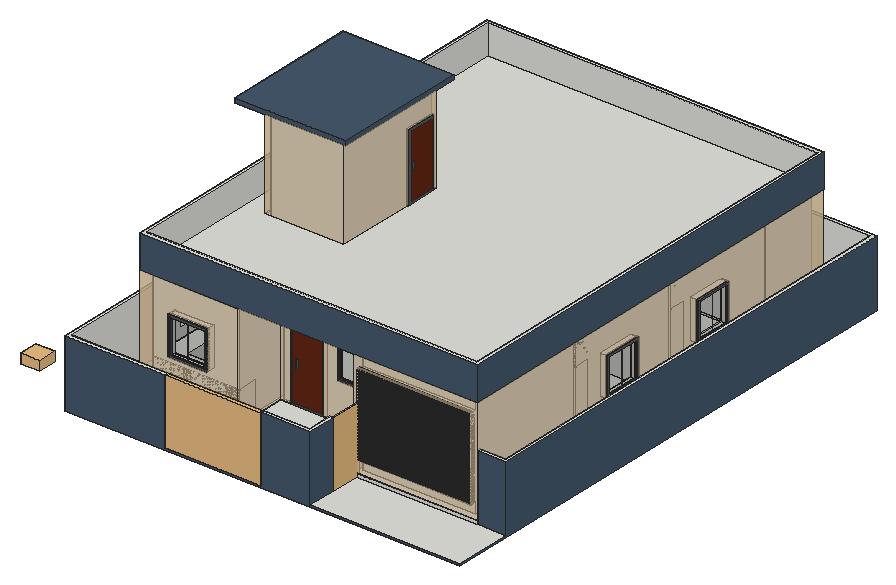
# SketchUp Ruby script. Lengths in inches.
U = 1.inch
M = Sketchup.active_model
def pt(a) = Geom::Point3d.new(a.map { |v| v * U })
def face(e, loops, mat)
  f = e.add_face(loops[0].map { |a| pt(a) })
  loops[1..].each { |l| e.add_face(l.map { |a| pt(a) }).erase! }
  f.material = f.back_material = mat if mat
  f
end
# faces: each face lists its corners as indices into pts; further lists are holes
def faces(e, pts, list, mat = nil) = list.each { |f| face(e, (f[0].is_a?(Array) ? f : [f]).map { |l| l.map { |i| pts[i] } }, mat) }
# xy, xz, yz: faces in a plane at the given z, y or x. An outline is a flat list of corners, or four numbers for a rectangle; further outlines are holes
def ring(l) = l.size == 4 ? [[l[0], l[1]], [l[2], l[1]], [l[2], l[3]], [l[0], l[3]]] : l.each_slice(2).to_a
def flat(e, list, mat, &to3) = list.each { |f| face(e, (f[0].is_a?(Array) ? f : [f]).map { |l| ring(l).map { |u, v| to3.(u, v) } }, mat) }
def xy(e, z, list, mat = nil) = flat(e, list, mat) { |x, y| [x, y, z] }
def xz(e, y, list, mat = nil) = flat(e, list, mat) { |x, z| [x, y, z] }
def yz(e, x, list, mat = nil) = flat(e, list, mat) { |y, z| [x, y, z] }
def lines(e, pts, list) = list.each { |a, b| e.add_line(pt(pts[a]), pt(pts[b])) }
# prism: a flat outline (further loops are holes) pulled along v
def prism(e, loops, v, mat = nil)
  f = face(e, loops, mat); d = Geom::Vector3d.new(v.map { |x| x * U })
  f.pushpull(f.normal.samedirection?(d) ? d.length : -d.length)
end
def box(e, o, s, mat = nil) = prism(e, [[o, [o[0] + s[0], o[1], o[2]], [o[0] + s[0], o[1] + s[1], o[2]], [o[0], o[1] + s[1], o[2]]]], [0, 0, s[2]], mat)
def at(x, y, z, deg = 0) = Geom::Transformation.translation(pt([x, y, z])) * Geom::Transformation.rotation(ORIGIN, Z_AXIS, deg.degrees)
def axes(o, x, y, z) = Geom::Transformation.new([*x, 0, *y, 0, *z, 0, *pt(o).to_a, 1])
def part(name) = M.definitions.add(name)
# library, detail: a bought-in or finely detailed component or shape, given as its bounding box
def library(name, o, s) = part(name).tap { |d| box(d.entities, o, s) }
def detail(e, o, s) = box(e.add_group.entities, o, s)
def put(e, d, t, mat = nil) = e.add_instance(d, t).tap { |i| i.material = mat if mat }
def group(e, t, mat = nil) = e.add_group.tap { |g| g.transformation = t; g.material = mat if mat }.entities
root = M.entities
M.materials.add("Chocolate White 001").color = [230, 202, 161]
M.materials["Chocolate White 001"].alpha = 0.6
M.materials.add("Glass Red 001").color = [0, 0, 0]
M.materials["Glass Red 001"].alpha = 0.1
M.materials.add("Metal Sandblasted Black 200cm").color = [86, 90, 95]
M.materials.add("Wall Paint Simple Reflective").color = [70, 89, 109]
M.materials.add("Wood Dark 02 100cm").color = [99, 39, 19]
M.materials.add("[Metal_Aluminum_Anodized]").color = [232, 200, 107]
c1 = library("gate 189k",[0,0,0],[125.98,4.8,118.11])
c2 = library("gate 130k",[0,-0.99,0],[39.37,1.78,88.58])
c3 = library("Dome Light",[-12,-12,0],[24,24,12])
c4 = part("Group\#3")
box(c4.entities,[-0.31,0,0],[0.31,22,44])
c5 = part("Group\#5")
box(c5.entities,[0,-0.31,0],[22,0.31,44])
c6 = part("Group\#13")
box(c6.entities,[0,0,0],[0.31,16,44])
c7 = part("Group\#15")
box(c7.entities,[0,0,0],[0.31,16.32,44])
c8 = part("Group\#19")
box(c8.entities,[0,0,0],[22,0.31,44])
c9 = part("Group\#7")
box(c9.entities,[0,-0.31,0],[32,0.31,2])
c10 = part("Group\#101")
box(c10.entities,[0,0,0],[0.31,22,44])
c11 = part("Group\#11")
box(c11.entities,[0,0,0],[0.31,32,2])
c12 = part("Group\#46")
box(c12.entities,[0,0,0],[0.71,39.5,117.71])
c13 = part("Group\#49")
box(c13.entities,[0,0,0],[0.71,20.65,34.58])
c14 = part("Group\#51")
g1 = group(c14.entities,at(12,0,0))
xy(g1,0,[[-12,0,0,84]])
xy(g1,1.96,[[-12,2.5,-2,81.5]])
xy(g1,94.04,[[-12,2.5,-2,81.5]])
xy(g1,96,[[-12,0,0,84]])
xz(g1,0,[[-12,0,0,96]])
xz(g1,2.5,[[-12,1.96,-2,94.04]])
xz(g1,81.5,[[-12,1.96,-2,94.04]])
xz(g1,84,[[-12,0,0,96]])
yz(g1,-12,[[[0,0,84,96],[2.5,1.96,81.5,94.04]]])
yz(g1,-2,[[2.5,1.96,81.5,94.04]])
yz(g1,0,[[0,0,84,96]])
put(g1,c12,axes([-12,42,1.96],[1,0,0],[0,1,0],[0,0,0.78232]))
put(g1,c12,axes([-12,2.5,1.96],[1,0,0],[0,1,0],[0,0,0.78232]))
g2 = group(c14.entities,at(0,0,96))
box(g2,[0,0,0],[12,84,36])
g3 = group(g2,at(0,21.05,0.71))
box(g3,[0,0,0],[0.71,20.95,34.58])
put(g2,c13,at(0,62.65,0.71))
put(g2,c13,at(0,42,0.71))
g4 = group(g2,at(0,0.1,0.71))
box(g4,[0,0,0],[0.71,20.95,34.58])
c15 = part("Group\#55")
box(c15.entities,[0,0,0],[12,36,6.5625])
c16 = part("Group\#64")
box(c16.entities,[0,0,0],[12,39.5,6.5625])
c17 = part("Group\#57")
box(c17.entities,[0,0,0],[12,36,6])
prism(root,[[[45,190,0],[69,190,0],[69,105,0],[153,105,0],[153,81,0],[45,81,0]]],[0,0,36])
prism(root,[[[45,454.5,0],[153,454.5,0],[153,430.5,0],[69,430.5,0],[69,370.5,0],[45,370.5,0]]],[0,0,36])
put(root,c1,axes([124.8,0,-4],[0.9476,0,0],[0,0.87,0],[0,0,0.69427]))
put(root,c2,axes([305.43,36,-4],[0,0.97964,0],[-1,0,0],[0,0,0.92569]),"[Metal_Aluminum_Anodized]")
put(root,c3,at(-71.79,47.18,1.82))
g5 = group(root,at(36,72,0))
xy(g5,0,[[[0,0,0,540,420,540,420,0,265.5,0,265.5,67,175.5,67,175.5,71.5,265.5,71.5,265.5,260,270,260,270,164,411,164,411,308,270,308,270,296,265.5,296,265.5,324.5,270,324.5,270,312.5,411,312.5,411,456.5,363,456.5,363,461,411,461,411,531,294,531,294,461,327,461,327,456.5,270,456.5,270,360.5,265.5,360.5,265.5,461,289.5,461,289.5,531,157.5,531,157.5,461,229.5,461,229.5,456.5,157.5,456.5,157.5,447,153,447,153,531,9,531,9,387,153,387,153,399,157.5,399,157.5,294,141,294,141,298.5,153,298.5,153,382.5,9,382.5,9,298.5,105,298.5,105,294,9,294,9,158.5,121.5,158.5,121.5,142,117,142,117,154,9,154,9,9,117,9,117,106,121.5,106,121.5,71.5,133.5,71.5,133.5,67,121.5,67,121.5,0],[270,9,411,159.5]]])
xy(g5,15.1875,[[270,0,411,9]])
xy(g5,36,[[270,99.5,294,99.5,294,135.5,387,135.5,387,99.5,411,99.5,411,159.5,270,159.5]])
xy(g5,48,[[36,0,84,9],[0,51.1875,9,99.1875],[193.375,67,241.375,71.5],[0,158.5,9,195.14],[411,201.4375,420,249.4375],
  [0,258,9,294],[411,342.15,420,390.15],[0,430.8125,9,478.8125],[64.4375,531,112.4375,540]])
xy(g5,72,[[0,324.8125,9,360.8125],[210.8125,531,246.8125,540],[339.375,531,375.375,540]])
xy(g5,96,[[36,0,84,9],[0,51.1875,9,99.1875],[133.5,67,175.5,71.5],[193.375,67,241.375,71.5],[117,106,121.5,142],
  [0,158.5,9,195.14],[411,201.4375,420,249.4375],[0,258,9,294],[265.5,260,270,296],[105,294,141,298.5],
  [265.5,324.5,270,360.5],[0,324.8125,9,360.8125],[411,342.15,420,390.15],[153,399,157.5,447],[0,430.8125,9,478.8125],
  [229.5,456.5,265.5,461],[327,456.5,363,461],[64.4375,531,112.4375,540],[210.8125,531,246.8125,540],[339.375,531,375.375,540]])
xy(g5,116.08,[[270,0,411,9]])
xy(g5,132,[[[0,0,121.5,0,121.5,67,265.5,67,265.5,0,420,0,420,540,0,540],[121.5,71.5,121.5,158.5,9,158.5,9,294,157.5,294,157.5,456.5,265.5,456.5,265.5,71.5],[270,9,411,159.5],[9,387,153,531],[270,164,411,308],[270,312.5,411,456.5],[9,9,117,154],[9,298.5,153,382.5],[157.5,461,289.5,531],[294,461,411,531]]])
xz(g5,0,[[[0,0,121.5,132],[36,48,84,96]],[[265.5,0,420,132],[270,15.1875,411,116.08]]],"Chocolate White 001")
xz(g5,9,[[[9,0,117,132],[36,48,84,96]],[270,0,411,15.1875],[270,116.08,411,132]])
xz(g5,51.1875,[[0,48,9,96]])
xz(g5,67,[[[121.5,0,133.5,0,133.5,96,175.5,96,175.5,0,265.5,0,265.5,132,121.5,132],[193.375,48,241.375,96]]],"Chocolate White 001")
xz(g5,71.5,[[[121.5,0,121.5,132,265.5,132,265.5,0,175.5,0,175.5,96,133.5,96,133.5,0],[193.375,48,241.375,96]]])
xz(g5,99.1875,[[0,48,9,96]])
xz(g5,99.5,[[270,0,294,36],[387,0,411,36]])
xz(g5,106,[[117,0,121.5,96]])
xz(g5,135.5,[[294,0,387,36]])
xz(g5,142,[[117,0,121.5,96]])
xz(g5,154,[[9,0,117,132]])
xz(g5,158.5,[[9,0,9,48,0,48,0,96,9,96,9,132,121.5,132,121.5,0]])
xz(g5,159.5,[[270,0,411,36],[270,36,411,132]])
xz(g5,164,[[270,0,411,132]])
xz(g5,195.14,[[0,48,9,96]])
xz(g5,201.4375,[[411,48,420,96]])
xz(g5,249.4375,[[411,48,420,96]])
xz(g5,258,[[0,48,9,96]])
xz(g5,260,[[265.5,0,270,96]])
xz(g5,294,[[9,0,105,0,105,96,141,96,141,0,157.5,0,157.5,132,9,132,9,96,0,96,0,48,9,48]])
xz(g5,296,[[265.5,0,270,96]])
xz(g5,298.5,[[9,0,9,132,153,132,153,0,141,0,141,96,105,96,105,0]])
xz(g5,308,[[270,0,411,132]])
xz(g5,312.5,[[270,0,411,132]])
xz(g5,324.5,[[265.5,0,270,96]])
xz(g5,324.8125,[[0,72,9,96]])
xz(g5,342.15,[[411,48,420,96]])
xz(g5,360.5,[[265.5,0,270,96]])
xz(g5,360.8125,[[0,72,9,96]])
xz(g5,382.5,[[9,0,153,132]])
xz(g5,387,[[9,0,153,132]])
xz(g5,390.15,[[411,48,420,96]])
xz(g5,399,[[153,0,157.5,96]])
xz(g5,430.8125,[[0,48,9,96]])
xz(g5,447,[[153,0,157.5,96]])
xz(g5,456.5,[[157.5,0,229.5,0,229.5,96,265.5,96,265.5,132,157.5,132],[270,0,327,0,327,96,363,96,363,0,411,0,411,132,270,132]])
xz(g5,461,[[157.5,0,157.5,132,289.5,132,289.5,0,265.5,0,265.5,96,229.5,96,229.5,0],[294,0,294,132,411,132,411,0,363,0,363,96,327,96,327,0]])
xz(g5,478.8125,[[0,48,9,96]])
xz(g5,531,[[[9,0,153,132],[64.4375,48,112.4375,96]],[[157.5,0,289.5,132],[210.8125,72,246.8125,96]],[[294,0,411,132],[339.375,72,375.375,96]]])
xz(g5,540,[[[0,0,420,132],[64.4375,48,112.4375,96],[339.375,72,375.375,96],[210.8125,72,246.8125,96]]],"Chocolate White 001")
yz(g5,0,[[[0,0,540,132],[430.8125,48,478.8125,96],[51.1875,48,99.1875,96],[158.5,48,195.14,96],[258,48,294,96],[324.8125,72,360.8125,96]]],"Chocolate White 001")
yz(g5,9,[[[9,0,154,132],[51.1875,48,99.1875,96]],[158.5,0,294,0,294,48,258,48,258,96,294,96,294,132,158.5,132,158.5,96,195.14,96,195.14,48,158.5,48],[[298.5,0,382.5,132],[324.8125,72,360.8125,96]],[[387,0,531,132],[430.8125,48,478.8125,96]]])
yz(g5,36,[[0,48,9,96]])
yz(g5,64.4375,[[531,48,540,96]])
yz(g5,84,[[0,48,9,96]])
yz(g5,105,[[294,0,298.5,96]])
yz(g5,112.4375,[[531,48,540,96]])
yz(g5,117,[[9,0,9,132,154,132,154,0,142,0,142,96,106,96,106,0]])
yz(g5,121.5,[[71.5,0,106,0,106,96,142,96,142,0,158.5,0,158.5,132,71.5,132]])
yz(g5,121.5,[[0,0,67,132]],"Chocolate White 001")
yz(g5,133.5,[[67,0,71.5,96]])
yz(g5,141,[[294,0,298.5,96]])
yz(g5,153,[[298.5,0,382.5,132],[387,0,387,132,531,132,531,0,447,0,447,96,399,96,399,0]])
yz(g5,157.5,[[294,0,399,0,399,96,447,96,447,0,456.5,0,456.5,132,294,132],[461,0,531,132]])
yz(g5,175.5,[[67,0,71.5,96]])
yz(g5,193.375,[[67,48,71.5,96]])
yz(g5,210.8125,[[531,72,540,96]])
yz(g5,229.5,[[456.5,0,461,96]])
yz(g5,241.375,[[67,48,71.5,96]])
yz(g5,246.8125,[[531,72,540,96]])
yz(g5,265.5,[[0,0,67,132],[71.5,0,71.5,132,456.5,132,456.5,96,461,96,461,0,360.5,0,360.5,96,324.5,96,324.5,0,296,0,296,96,260,96,260,0]])
yz(g5,270,[[9,0,99.5,0,99.5,36,159.5,36,159.5,132,9,132,9,116.08,0,116.08,0,15.1875,9,15.1875],[99.5,0,159.5,36],[164,0,260,0,260,96,296,96,296,0,308,0,308,132,164,132],[312.5,0,324.5,0,324.5,96,360.5,96,360.5,0,456.5,0,456.5,132,312.5,132]])
yz(g5,289.5,[[461,0,531,132]])
yz(g5,294,[[99.5,0,135.5,36],[461,0,531,132]])
yz(g5,327,[[456.5,0,461,96]])
yz(g5,339.375,[[531,72,540,96]])
yz(g5,363,[[456.5,0,461,96]])
yz(g5,375.375,[[531,72,540,96]])
yz(g5,387,[[99.5,0,135.5,36]])
yz(g5,411,[[9,0,9,15.1875,0,15.1875,0,116.08,9,116.08,9,132,159.5,132,159.5,36,99.5,36,99.5,0],[99.5,0,159.5,36],[[164,0,308,132],[201.4375,48,249.4375,96]],[[312.5,0,456.5,132],[342.15,48,390.15,96]],[461,0,531,132]])
yz(g5,420,[[[0,0,540,132],[201.4375,48,249.4375,96],[342.15,48,390.15,96]]],"Chocolate White 001")
g6 = group(g5,at(420,201.4375,48))
prism(g6,[[[1.5,48,0],[1.5,48,48],[1.5,0,48],[1.5,0,0]],[[1.5,46,46],[1.5,46,2],[1.5,2,2],[1.5,2,46]]],[-3,0,0],"Metal Sandblasted Black 200cm")
put(g6,c4,at(0,2,2),"Glass Red 001")
put(g6,c4,at(0.375,24,2),"Glass Red 001")
g7 = group(g5,at(420,342.15,48))
prism(g7,[[[1.5,48,0],[1.5,48,48],[1.5,0,48],[1.5,0,0]],[[1.5,46,46],[1.5,46,2],[1.5,2,2],[1.5,2,46]]],[-3,0,0],"Metal Sandblasted Black 200cm")
put(g7,c4,at(0,2,2),"Glass Red 001")
put(g7,c4,at(0.375,24,2),"Glass Red 001")
g8 = group(g5,at(64.4375,540,48))
prism(g8,[[[48,1.5,0],[0,1.5,0],[0,1.5,48],[48,1.5,48]],[[46,1.5,46],[2,1.5,46],[2,1.5,2],[46,1.5,2]]],[0,-3,0],"Metal Sandblasted Black 200cm")
put(g8,c5,at(24,-0.125,2),"Glass Red 001")
put(g8,c5,at(2,0.19,2),"Glass Red 001")
g9 = group(g5,at(0,258,48))
prism(g9,[[[-1.5,0,0],[-1.5,0,48],[-1.5,36,48],[-1.5,36,0]],[[-1.5,2,46],[-1.5,2,2],[-1.5,34,2],[-1.5,34,46]]],[3,0,0],"Metal Sandblasted Black 200cm")
put(g9,c6,at(-0.0625,18,2),"Glass Red 001")
put(g9,c6,at(-0.38,2,2),"Glass Red 001")
g10 = group(g5,at(0,158.5,48))
prism(g10,[[[-1.5,0,0],[-1.5,0,48],[-1.5,36.64,48],[-1.5,36.64,0]],[[-1.5,2,2],[-1.5,34.64,2],[-1.5,34.64,46],[-1.5,2,46]]],[3,0,0],"Metal Sandblasted Black 200cm")
put(g10,c7,at(0.25,18.32,2),"Glass Red 001")
put(g10,c7,at(-0.06,2,2),"Glass Red 001")
g11 = group(g5,at(36,0,48))
prism(g11,[[[48,-1.5,0],[48,-1.5,48],[0,-1.5,48],[0,-1.5,0]],[[46,-1.5,2],[2,-1.5,2],[2,-1.5,46],[46,-1.5,46]]],[0,3,0],"Metal Sandblasted Black 200cm")
g12 = group(g11,at(2,0.25,2))
box(g12,[0,0,0],[22,0.31,44],"Glass Red 001")
g13 = group(g11,at(24,-0.06,2))
box(g13,[0,0,0],[22,0.31,44],"Glass Red 001")
g14 = group(g5,at(193.375,67,48))
prism(g14,[[[0,-1.5,0],[48,-1.5,0],[48,-1.5,48],[0,-1.5,48]],[[46,-1.5,46],[46,-1.5,2],[2,-1.5,2],[2,-1.5,46]]],[0,3,0],"Metal Sandblasted Black 200cm")
put(g14,c8,at(2,0.25,2),"Glass Red 001")
put(g14,c8,at(24,-0.06,2),"Glass Red 001")
g15 = group(g5,at(105,294,0))
prism(g15,[[[36,0,0],[36,0,96],[0,0,96],[0,0,0]],[[2,0,94],[34,0,94],[34,0,2],[2,0,2]]],[0,2.5,0])
g16 = group(g15,at(2,0,2))
box(g16,[0,0,0],[32,0.71,92])
g17 = group(g16,at(4.04,0,47.62))
box(g17,[0,-0.4375,0],[1.5,0.4375,8.75])
g18 = group(g5,at(265.5,260,0))
prism(g18,[[[0,0,0],[0,0,96],[0,36,96],[0,36,0]],[[0,2,94],[0,2,2],[0,34,2],[0,34,94]]],[2.5,0,0])
g19 = group(g18,at(0,2,2))
box(g19,[0,0,0],[0.71,32,92])
g20 = group(g19,at(0,28.94,45.79))
box(g20,[-0.375,-0.875,-2.25],[0.375,0.875,7.1875])
g21 = group(g5,at(265.5,324.5,0))
prism(g21,[[[0,0,0],[0,0,96],[0,36,96],[0,36,0]],[[0,2,94],[0,2,2],[0,34,2],[0,34,94]]],[2.5,0,0])
g22 = group(g21,at(0,2,2))
box(g22,[0,0,0],[0.71,32,92])
g23 = group(g22,at(0,29.6,45.12))
box(g23,[-0.5,-1.5,0],[0.5,1.5,9.25])
g24 = group(g5,at(327,456.5,0))
prism(g24,[[[36,0,0],[36,0,96],[0,0,96],[0,0,0]],[[2,0,2],[2,0,94],[34,0,94],[34,0,2]]],[0,2.5,0])
g25 = group(g24,at(2,0,2))
box(g25,[0,0,0],[32,0.71,92])
g26 = group(g25,at(4.72,0,44.53))
box(g26,[0,-0.8125,0],[1.625,0.8125,8.625])
g27 = group(g5,at(229.5,456.5,0))
prism(g27,[[[36,0,0],[36,0,96],[0,0,96],[0,0,0]],[[2,0,94],[34,0,94],[34,0,2],[2,0,2]]],[0,2.5,0])
g28 = group(g27,at(2,0,2))
box(g28,[0,0,0],[32,0.71,92])
g29 = group(g28,at(5.2,0,51.08))
box(g29,[0,-0.5,0],[1.3125,0.5,8])
g30 = group(g5,at(157.5,399,0))
prism(g30,[[[0,48,0],[0,48,96],[0,0,96],[0,0,0]],[[0,46,2],[0,2,2],[0,2,94],[0,46,94]]],[-2.5,0,0])
g31 = group(g30,at(0,2,2))
box(g31,[-0.71,0,0],[0.71,44,92])
g32 = group(g31,at(0,3.72,42.1875))
box(g32,[0,0,0],[0.875,2.3125,11.125])
g33 = group(root,at(375.375,612,72))
prism(g33,[[[0,1.5,24],[36,1.5,24],[36,1.5,0],[0,1.5,0]],[[34,1.5,2],[34,1.5,22],[2,1.5,22],[2,1.5,2]]],[0,-3,0],"Metal Sandblasted Black 200cm")
put(g33,c9,at(2,1.5,20),"Glass Red 001")
put(g33,c9,at(2,1.5,17),"Glass Red 001")
put(g33,c9,at(2,1.5,14),"Glass Red 001")
put(g33,c9,at(2,1.5,11),"Glass Red 001")
put(g33,c9,at(2,1.5,8),"Glass Red 001")
put(g33,c9,at(2,1.5,5),"Glass Red 001")
put(g33,c9,at(2,1.5,2),"Glass Red 001")
g34 = group(root,at(246.8125,612,72))
prism(g34,[[[0,1.5,24],[36,1.5,24],[36,1.5,0],[0,1.5,0]],[[34,1.5,2],[34,1.5,22],[2,1.5,22],[2,1.5,2]]],[0,-3,0],"Metal Sandblasted Black 200cm")
put(g34,c9,at(2,1.5,20),"Glass Red 001")
put(g34,c9,at(2,1.5,17),"Glass Red 001")
put(g34,c9,at(2,1.5,14),"Glass Red 001")
put(g34,c9,at(2,1.5,11),"Glass Red 001")
put(g34,c9,at(2,1.5,8),"Glass Red 001")
put(g34,c9,at(2,1.5,5),"Glass Red 001")
put(g34,c9,at(2,1.5,2),"Glass Red 001")
g35 = group(root,at(36,502.8125,48))
prism(g35,[[[-1.5,48,0],[-1.5,0,0],[-1.5,0,48],[-1.5,48,48]],[[-1.5,2,2],[-1.5,46,2],[-1.5,46,46],[-1.5,2,46]]],[3,0,0],"Metal Sandblasted Black 200cm")
put(g35,c10,at(0.3125,24,2),"Glass Red 001")
put(g35,c10,at(0,2,2),"Glass Red 001")
g36 = group(root,at(36,396.8125,72))
prism(g36,[[[-1.5,36,24],[-1.5,36,0],[-1.5,0,0],[-1.5,0,24]],[[-1.5,2,2],[-1.5,34,2],[-1.5,34,22],[-1.5,2,22]]],[3,0,0],"Metal Sandblasted Black 200cm")
put(g36,c11,at(-1.5,2,20),"Glass Red 001")
put(g36,c11,at(-1.5,2,17),"Glass Red 001")
put(g36,c11,at(-1.5,2,14),"Glass Red 001")
put(g36,c11,at(-1.5,2,11),"Glass Red 001")
put(g36,c11,at(-1.5,2,8),"Glass Red 001")
put(g36,c11,at(-1.5,2,5),"Glass Red 001")
put(g36,c11,at(-1.5,2,2),"Glass Red 001")
g37 = group(root,at(36,123.1875,48))
prism(g37,[[[-1.5,48,0],[-1.5,0,0],[-1.5,0,48],[-1.5,48,48]],[[-1.5,2,2],[-1.5,46,2],[-1.5,46,46],[-1.5,2,46]]],[3,0,0],"Metal Sandblasted Black 200cm")
g38 = group(g37,at(0.3125,24,2))
box(g38,[0,0,0],[0.31,22,44],"Glass Red 001")
put(g37,c10,at(0,2,2),"Glass Red 001")
g39 = group(root,at(157.5,178,0))
prism(g39,[[[0,36,96],[0,0,96],[0,0,0],[0,36,0]],[[0,34,2],[0,2,2],[0,2,94],[0,34,94]]],[-2.5,0,0])
g40 = group(g39,at(0,2,2))
box(g40,[-0.71,0,0],[0.71,32,92])
g41 = group(g40,at(0,4.56,43.3))
box(g41,[0,0,0],[0.625,2.125,13.125])
g42 = group(root,at(169.5,139,0))
prism(g42,[[[0,0,0],[42,0,0],[42,0,96],[0,0,96]],[[2,0,2],[2,0,94],[40,0,94],[40,0,2]]],[0,2.5,0],"Metal Sandblasted Black 200cm")
g43 = group(g42,at(2,0,2))
xy(g43,0,[[0,0,38,0.71]])
xy(g43,92,[[0,0,38,0.71]])
xz(g43,0,[[0,0,38,92]],"Wood Dark 02 100cm")
xz(g43,0.71,[[0,0,38,92]])
yz(g43,0,[[0,0,0.71,92]])
yz(g43,38,[[0,0,0.71,92]])
g44 = group(g43,at(4.7,0,40.24),"Metal Sandblasted Black 200cm")
xy(g44,0,[[0,-0.6875,1.9375,0]])
xy(g44,10.0625,[[0,-0.6875,1.9375,0]])
xz(g44,-0.6875,[[0,0,1.9375,10.0625]],"Metal Sandblasted Black 200cm")
xz(g44,0,[[0,0,1.9375,10.0625]],"Metal Sandblasted Black 200cm")
yz(g44,0,[[-0.6875,0,0,10.0625]],"Metal Sandblasted Black 200cm")
yz(g44,1.9375,[[-0.6875,0,0,10.0625]],"Metal Sandblasted Black 200cm")
g45 = group(root,at(447,72.9,13.7))
prism(g45,[[[0,4.2,1.125],[0,4.42,1.67],[0,4.5,2.25],[0,4.42,2.83],[0,4.2,3.375],[0,3.84,3.84],[0,3.375,4.2],[0,2.83,4.42],[0,2.25,4.5],[0,1.67,4.42],[0,1.125,4.2],[0,0.66,3.84],[0,0.3,3.375],[0,0.08,2.83],[0,0,2.25],[0,0.08,1.67],[0,0.3,1.125],[0,0.66,0.66],[0,1.125,0.3],[0,1.67,0.08],[0,2.25,0],[0,2.83,0.08],[0,3.375,0.3],[0,3.84,0.66]]],[-141,0,0],"Metal Sandblasted Black 200cm")
g46 = group(root,at(447,72.9,16.98))
prism(g46,[[[0,4.2,1.125],[0,4.42,1.67],[0,4.5,2.25],[0,4.42,2.83],[0,4.2,3.375],[0,3.84,3.84],[0,3.375,4.2],[0,2.83,4.42],[0,2.25,4.5],[0,1.67,4.42],[0,1.125,4.2],[0,0.66,3.84],[0,0.3,3.375],[0,0.08,2.83],[0,0,2.25],[0,0.08,1.67],[0,0.3,1.125],[0,0.66,0.66],[0,1.125,0.3],[0,1.67,0.08],[0,2.25,0],[0,2.83,0.08],[0,3.375,0.3],[0,3.84,0.66]]],[-141,0,0],"Metal Sandblasted Black 200cm")
g47 = group(root,at(447,72.9,20.27))
prism(g47,[[[0,4.2,1.125],[0,4.42,1.67],[0,4.5,2.25],[0,4.42,2.83],[0,4.2,3.375],[0,3.84,3.84],[0,3.375,4.2],[0,2.83,4.42],[0,2.25,4.5],[0,1.67,4.42],[0,1.125,4.2],[0,0.66,3.84],[0,0.3,3.375],[0,0.08,2.83],[0,0,2.25],[0,0.08,1.67],[0,0.3,1.125],[0,0.66,0.66],[0,1.125,0.3],[0,1.67,0.08],[0,2.25,0],[0,2.83,0.08],[0,3.375,0.3],[0,3.84,0.66]]],[-141,0,0],"Metal Sandblasted Black 200cm")
g48 = group(root,at(447,72.9,23.56))
prism(g48,[[[0,4.2,1.125],[0,4.42,1.67],[0,4.5,2.25],[0,4.42,2.83],[0,4.2,3.375],[0,3.84,3.84],[0,3.375,4.2],[0,2.83,4.42],[0,2.25,4.5],[0,1.67,4.42],[0,1.125,4.2],[0,0.66,3.84],[0,0.3,3.375],[0,0.08,2.83],[0,0,2.25],[0,0.08,1.67],[0,0.3,1.125],[0,0.66,0.66],[0,1.125,0.3],[0,1.67,0.08],[0,2.25,0],[0,2.83,0.08],[0,3.375,0.3],[0,3.84,0.66]]],[-141,0,0],"Metal Sandblasted Black 200cm")
g49 = group(root,at(447,72.9,26.85))
prism(g49,[[[0,4.2,1.125],[0,4.42,1.67],[0,4.5,2.25],[0,4.42,2.83],[0,4.2,3.375],[0,3.84,3.84],[0,3.375,4.2],[0,2.83,4.42],[0,2.25,4.5],[0,1.67,4.42],[0,1.125,4.2],[0,0.66,3.84],[0,0.3,3.375],[0,0.08,2.83],[0,0,2.25],[0,0.08,1.67],[0,0.3,1.125],[0,0.66,0.66],[0,1.125,0.3],[0,1.67,0.08],[0,2.25,0],[0,2.83,0.08],[0,3.375,0.3],[0,3.84,0.66]]],[-141,0,0],"Metal Sandblasted Black 200cm")
g50 = group(root,at(447,72.9,30.13))
prism(g50,[[[0,4.2,1.125],[0,4.42,1.67],[0,4.5,2.25],[0,4.42,2.83],[0,4.2,3.375],[0,3.84,3.84],[0,3.375,4.2],[0,2.83,4.42],[0,2.25,4.5],[0,1.67,4.42],[0,1.125,4.2],[0,0.66,3.84],[0,0.3,3.375],[0,0.08,2.83],[0,0,2.25],[0,0.08,1.67],[0,0.3,1.125],[0,0.66,0.66],[0,1.125,0.3],[0,1.67,0.08],[0,2.25,0],[0,2.83,0.08],[0,3.375,0.3],[0,3.84,0.66]]],[-141,0,0],"Metal Sandblasted Black 200cm")
g51 = group(root,at(447,72.9,33.42))
prism(g51,[[[0,4.2,1.125],[0,4.42,1.67],[0,4.5,2.25],[0,4.42,2.83],[0,4.2,3.375],[0,3.84,3.84],[0,3.375,4.2],[0,2.83,4.42],[0,2.25,4.5],[0,1.67,4.42],[0,1.125,4.2],[0,0.66,3.84],[0,0.3,3.375],[0,0.08,2.83],[0,0,2.25],[0,0.08,1.67],[0,0.3,1.125],[0,0.66,0.66],[0,1.125,0.3],[0,1.67,0.08],[0,2.25,0],[0,2.83,0.08],[0,3.375,0.3],[0,3.84,0.66]]],[-141,0,0],"Metal Sandblasted Black 200cm")
g52 = group(root,at(447,72.9,36.71))
prism(g52,[[[0,4.2,1.125],[0,4.42,1.67],[0,4.5,2.25],[0,4.42,2.83],[0,4.2,3.375],[0,3.84,3.84],[0,3.375,4.2],[0,2.83,4.42],[0,2.25,4.5],[0,1.67,4.42],[0,1.125,4.2],[0,0.66,3.84],[0,0.3,3.375],[0,0.08,2.83],[0,0,2.25],[0,0.08,1.67],[0,0.3,1.125],[0,0.66,0.66],[0,1.125,0.3],[0,1.67,0.08],[0,2.25,0],[0,2.83,0.08],[0,3.375,0.3],[0,3.84,0.66]]],[-141,0,0],"Metal Sandblasted Black 200cm")
g53 = group(root,at(447,72.9,40))
prism(g53,[[[0,4.2,1.125],[0,4.42,1.67],[0,4.5,2.25],[0,4.42,2.83],[0,4.2,3.375],[0,3.84,3.84],[0,3.375,4.2],[0,2.83,4.42],[0,2.25,4.5],[0,1.67,4.42],[0,1.125,4.2],[0,0.66,3.84],[0,0.3,3.375],[0,0.08,2.83],[0,0,2.25],[0,0.08,1.67],[0,0.3,1.125],[0,0.66,0.66],[0,1.125,0.3],[0,1.67,0.08],[0,2.25,0],[0,2.83,0.08],[0,3.375,0.3],[0,3.84,0.66]]],[-141,0,0],"Metal Sandblasted Black 200cm")
g54 = group(root,at(447,72.9,43.28))
prism(g54,[[[0,4.2,1.125],[0,4.42,1.67],[0,4.5,2.25],[0,4.42,2.83],[0,4.2,3.375],[0,3.84,3.84],[0,3.375,4.2],[0,2.83,4.42],[0,2.25,4.5],[0,1.67,4.42],[0,1.125,4.2],[0,0.66,3.84],[0,0.3,3.375],[0,0.08,2.83],[0,0,2.25],[0,0.08,1.67],[0,0.3,1.125],[0,0.66,0.66],[0,1.125,0.3],[0,1.67,0.08],[0,2.25,0],[0,2.83,0.08],[0,3.375,0.3],[0,3.84,0.66]]],[-141,0,0],"Metal Sandblasted Black 200cm")
g55 = group(root,at(447,72.9,46.57))
prism(g55,[[[0,4.2,1.125],[0,4.42,1.67],[0,4.5,2.25],[0,4.42,2.83],[0,4.2,3.375],[0,3.84,3.84],[0,3.375,4.2],[0,2.83,4.42],[0,2.25,4.5],[0,1.67,4.42],[0,1.125,4.2],[0,0.66,3.84],[0,0.3,3.375],[0,0.08,2.83],[0,0,2.25],[0,0.08,1.67],[0,0.3,1.125],[0,0.66,0.66],[0,1.125,0.3],[0,1.67,0.08],[0,2.25,0],[0,2.83,0.08],[0,3.375,0.3],[0,3.84,0.66]]],[-141,0,0],"Metal Sandblasted Black 200cm")
g56 = group(root,at(447,72.9,49.86))
prism(g56,[[[0,4.2,1.125],[0,4.42,1.67],[0,4.5,2.25],[0,4.42,2.83],[0,4.2,3.375],[0,3.84,3.84],[0,3.375,4.2],[0,2.83,4.42],[0,2.25,4.5],[0,1.67,4.42],[0,1.125,4.2],[0,0.66,3.84],[0,0.3,3.375],[0,0.08,2.83],[0,0,2.25],[0,0.08,1.67],[0,0.3,1.125],[0,0.66,0.66],[0,1.125,0.3],[0,1.67,0.08],[0,2.25,0],[0,2.83,0.08],[0,3.375,0.3],[0,3.84,0.66]]],[-141,0,0],"Metal Sandblasted Black 200cm")
g57 = group(root,at(447,72.9,53.15))
prism(g57,[[[0,4.2,1.125],[0,4.42,1.67],[0,4.5,2.25],[0,4.42,2.83],[0,4.2,3.375],[0,3.84,3.84],[0,3.375,4.2],[0,2.83,4.42],[0,2.25,4.5],[0,1.67,4.42],[0,1.125,4.2],[0,0.66,3.84],[0,0.3,3.375],[0,0.08,2.83],[0,0,2.25],[0,0.08,1.67],[0,0.3,1.125],[0,0.66,0.66],[0,1.125,0.3],[0,1.67,0.08],[0,2.25,0],[0,2.83,0.08],[0,3.375,0.3],[0,3.84,0.66]]],[-141,0,0],"Metal Sandblasted Black 200cm")
g58 = group(root,at(447,72.9,56.43))
prism(g58,[[[0,4.2,1.125],[0,4.42,1.67],[0,4.5,2.25],[0,4.42,2.83],[0,4.2,3.375],[0,3.84,3.84],[0,3.375,4.2],[0,2.83,4.42],[0,2.25,4.5],[0,1.67,4.42],[0,1.125,4.2],[0,0.66,3.84],[0,0.3,3.375],[0,0.08,2.83],[0,0,2.25],[0,0.08,1.67],[0,0.3,1.125],[0,0.66,0.66],[0,1.125,0.3],[0,1.67,0.08],[0,2.25,0],[0,2.83,0.08],[0,3.375,0.3],[0,3.84,0.66]]],[-141,0,0],"Metal Sandblasted Black 200cm")
g59 = group(root,at(447,72.9,59.72))
prism(g59,[[[0,4.2,1.125],[0,4.42,1.67],[0,4.5,2.25],[0,4.42,2.83],[0,4.2,3.375],[0,3.84,3.84],[0,3.375,4.2],[0,2.83,4.42],[0,2.25,4.5],[0,1.67,4.42],[0,1.125,4.2],[0,0.66,3.84],[0,0.3,3.375],[0,0.08,2.83],[0,0,2.25],[0,0.08,1.67],[0,0.3,1.125],[0,0.66,0.66],[0,1.125,0.3],[0,1.67,0.08],[0,2.25,0],[0,2.83,0.08],[0,3.375,0.3],[0,3.84,0.66]]],[-141,0,0],"Metal Sandblasted Black 200cm")
g60 = group(root,at(447,72.9,63.01))
prism(g60,[[[0,4.2,1.125],[0,4.42,1.67],[0,4.5,2.25],[0,4.42,2.83],[0,4.2,3.375],[0,3.84,3.84],[0,3.375,4.2],[0,2.83,4.42],[0,2.25,4.5],[0,1.67,4.42],[0,1.125,4.2],[0,0.66,3.84],[0,0.3,3.375],[0,0.08,2.83],[0,0,2.25],[0,0.08,1.67],[0,0.3,1.125],[0,0.66,0.66],[0,1.125,0.3],[0,1.67,0.08],[0,2.25,0],[0,2.83,0.08],[0,3.375,0.3],[0,3.84,0.66]]],[-141,0,0],"Metal Sandblasted Black 200cm")
g61 = group(root,at(447,72.9,66.3))
prism(g61,[[[0,4.2,1.125],[0,4.42,1.67],[0,4.5,2.25],[0,4.42,2.83],[0,4.2,3.375],[0,3.84,3.84],[0,3.375,4.2],[0,2.83,4.42],[0,2.25,4.5],[0,1.67,4.42],[0,1.125,4.2],[0,0.66,3.84],[0,0.3,3.375],[0,0.08,2.83],[0,0,2.25],[0,0.08,1.67],[0,0.3,1.125],[0,0.66,0.66],[0,1.125,0.3],[0,1.67,0.08],[0,2.25,0],[0,2.83,0.08],[0,3.375,0.3],[0,3.84,0.66]]],[-141,0,0],"Metal Sandblasted Black 200cm")
g62 = group(root,at(447,72.9,69.58))
prism(g62,[[[0,4.2,1.125],[0,4.42,1.67],[0,4.5,2.25],[0,4.42,2.83],[0,4.2,3.375],[0,3.84,3.84],[0,3.375,4.2],[0,2.83,4.42],[0,2.25,4.5],[0,1.67,4.42],[0,1.125,4.2],[0,0.66,3.84],[0,0.3,3.375],[0,0.08,2.83],[0,0,2.25],[0,0.08,1.67],[0,0.3,1.125],[0,0.66,0.66],[0,1.125,0.3],[0,1.67,0.08],[0,2.25,0],[0,2.83,0.08],[0,3.375,0.3],[0,3.84,0.66]]],[-141,0,0],"Metal Sandblasted Black 200cm")
g63 = group(root,at(447,72.9,72.87))
prism(g63,[[[0,4.2,1.125],[0,4.42,1.67],[0,4.5,2.25],[0,4.42,2.83],[0,4.2,3.375],[0,3.84,3.84],[0,3.375,4.2],[0,2.83,4.42],[0,2.25,4.5],[0,1.67,4.42],[0,1.125,4.2],[0,0.66,3.84],[0,0.3,3.375],[0,0.08,2.83],[0,0,2.25],[0,0.08,1.67],[0,0.3,1.125],[0,0.66,0.66],[0,1.125,0.3],[0,1.67,0.08],[0,2.25,0],[0,2.83,0.08],[0,3.375,0.3],[0,3.84,0.66]]],[-141,0,0],"Metal Sandblasted Black 200cm")
g64 = group(root,at(447,72.9,76.16))
prism(g64,[[[0,4.2,1.125],[0,4.42,1.67],[0,4.5,2.25],[0,4.42,2.83],[0,4.2,3.375],[0,3.84,3.84],[0,3.375,4.2],[0,2.83,4.42],[0,2.25,4.5],[0,1.67,4.42],[0,1.125,4.2],[0,0.66,3.84],[0,0.3,3.375],[0,0.08,2.83],[0,0,2.25],[0,0.08,1.67],[0,0.3,1.125],[0,0.66,0.66],[0,1.125,0.3],[0,1.67,0.08],[0,2.25,0],[0,2.83,0.08],[0,3.375,0.3],[0,3.84,0.66]]],[-141,0,0],"Metal Sandblasted Black 200cm")
g65 = group(root,at(447,72.9,79.45))
prism(g65,[[[0,4.2,1.125],[0,4.42,1.67],[0,4.5,2.25],[0,4.42,2.83],[0,4.2,3.375],[0,3.84,3.84],[0,3.375,4.2],[0,2.83,4.42],[0,2.25,4.5],[0,1.67,4.42],[0,1.125,4.2],[0,0.66,3.84],[0,0.3,3.375],[0,0.08,2.83],[0,0,2.25],[0,0.08,1.67],[0,0.3,1.125],[0,0.66,0.66],[0,1.125,0.3],[0,1.67,0.08],[0,2.25,0],[0,2.83,0.08],[0,3.375,0.3],[0,3.84,0.66]]],[-141,0,0],"Metal Sandblasted Black 200cm")
g66 = group(root,at(447,72.9,82.73))
yz(g66,-141,[[2.25,0,1.67,0.08,1.125,0.3,0.66,0.66,0.3,1.125,0.08,1.67,0,2.25,0.08,2.83,0.3,3.375,0.66,3.84,1.125,4.2,1.67,4.42,2.25,4.5,2.83,4.42,3.375,4.2,3.84,3.84,4.2,3.375,4.42,2.83,4.5,2.25,4.42,1.67,4.2,1.125,3.84,0.66,3.375,0.3,2.83,0.08]])
yz(g66,0,[[2.25,0,2.83,0.08,3.375,0.3,3.84,0.66,4.2,1.125,4.42,1.67,4.5,2.25,4.42,2.83,4.2,3.375,3.84,3.84,3.375,4.2,2.83,4.42,2.25,4.5,1.67,4.42,1.125,4.2,0.66,3.84,0.3,3.375,0.08,2.83,0,2.25,0.08,1.67,0.3,1.125,0.66,0.66,1.125,0.3,1.67,0.08]])
p = [[0,2.25,0],[0,1.67,0.08],[-141,1.67,0.08],[-141,2.25,0],[0,2.83,0.08],[-141,2.83,0.08],
  [0,1.125,0.3],[-141,1.125,0.3],[0,3.375,0.3],[-141,3.375,0.3],[0,0.66,0.66],[-141,0.66,0.66],
  [0,3.84,0.66],[-141,3.84,0.66],[0,0.3,1.125],[-141,0.3,1.125],[0,4.2,1.125],[-141,4.2,1.125],
  [0,0.08,1.67],[-141,0.08,1.67],[0,4.42,1.67],[-141,4.42,1.67],[0,0,2.25],[-141,0,2.25],
  [0,4.5,2.25],[-141,4.5,2.25],[0,0.08,2.83],[-141,0.08,2.83],[0,4.42,2.83],[-141,4.42,2.83],
  [0,0.3,3.375],[-141,0.3,3.375],[0,4.2,3.375],[-141,4.2,3.375],[0,0.66,3.84],[-141,0.66,3.84],
  [0,3.84,3.84],[-141,3.84,3.84],[0,1.125,4.2],[-141,1.125,4.2],[0,3.375,4.2],[-141,3.375,4.2],
  [0,1.67,4.42],[-141,1.67,4.42],[0,2.83,4.42],[-141,2.83,4.42],[0,2.25,4.5],[-141,2.25,4.5]]
faces(g66,p,[[0,1,2,3],[4,0,3,5],[1,6,7,2],[8,4,5,9],[6,10,11,7],[12,8,9,13],[10,14,15,11],[16,12,13,17],
  [14,18,19,15],[20,16,17,21],[18,22,23,19],[24,20,21,25],[22,26,27,23],[28,24,25,29],[26,30,31,27],[32,28,29,33],
  [30,34,35,31],[36,32,33,37],[34,38,39,35],[40,36,37,41],[38,42,43,39],[44,40,41,45],[42,46,47,43],[46,44,45,47]],"Metal Sandblasted Black 200cm")
g67 = group(root,at(447,72.9,86.02))
prism(g67,[[[0,4.2,1.125],[0,4.42,1.67],[0,4.5,2.25],[0,4.42,2.83],[0,4.2,3.375],[0,3.84,3.84],[0,3.375,4.2],[0,2.83,4.42],[0,2.25,4.5],[0,1.67,4.42],[0,1.125,4.2],[0,0.66,3.84],[0,0.3,3.375],[0,0.08,2.83],[0,0,2.25],[0,0.08,1.67],[0,0.3,1.125],[0,0.66,0.66],[0,1.125,0.3],[0,1.67,0.08],[0,2.25,0],[0,2.83,0.08],[0,3.375,0.3],[0,3.84,0.66]]],[-141,0,0],"Metal Sandblasted Black 200cm")
g68 = group(root,at(447,72.9,89.31))
prism(g68,[[[0,4.2,1.125],[0,4.42,1.67],[0,4.5,2.25],[0,4.42,2.83],[0,4.2,3.375],[0,3.84,3.84],[0,3.375,4.2],[0,2.83,4.42],[0,2.25,4.5],[0,1.67,4.42],[0,1.125,4.2],[0,0.66,3.84],[0,0.3,3.375],[0,0.08,2.83],[0,0,2.25],[0,0.08,1.67],[0,0.3,1.125],[0,0.66,0.66],[0,1.125,0.3],[0,1.67,0.08],[0,2.25,0],[0,2.83,0.08],[0,3.375,0.3],[0,3.84,0.66]]],[-141,0,0],"Metal Sandblasted Black 200cm")
g69 = group(root,at(447,72.9,92.6))
prism(g69,[[[0,4.2,1.125],[0,4.42,1.67],[0,4.5,2.25],[0,4.42,2.83],[0,4.2,3.375],[0,3.84,3.84],[0,3.375,4.2],[0,2.83,4.42],[0,2.25,4.5],[0,1.67,4.42],[0,1.125,4.2],[0,0.66,3.84],[0,0.3,3.375],[0,0.08,2.83],[0,0,2.25],[0,0.08,1.67],[0,0.3,1.125],[0,0.66,0.66],[0,1.125,0.3],[0,1.67,0.08],[0,2.25,0],[0,2.83,0.08],[0,3.375,0.3],[0,3.84,0.66]]],[-141,0,0],"Metal Sandblasted Black 200cm")
g70 = group(root,at(447,72.9,95.88))
prism(g70,[[[0,4.2,1.125],[0,4.42,1.67],[0,4.5,2.25],[0,4.42,2.83],[0,4.2,3.375],[0,3.84,3.84],[0,3.375,4.2],[0,2.83,4.42],[0,2.25,4.5],[0,1.67,4.42],[0,1.125,4.2],[0,0.66,3.84],[0,0.3,3.375],[0,0.08,2.83],[0,0,2.25],[0,0.08,1.67],[0,0.3,1.125],[0,0.66,0.66],[0,1.125,0.3],[0,1.67,0.08],[0,2.25,0],[0,2.83,0.08],[0,3.375,0.3],[0,3.84,0.66]]],[-141,0,0],"Metal Sandblasted Black 200cm")
g71 = group(root,at(447,72.9,99.17))
prism(g71,[[[0,4.2,1.125],[0,4.42,1.67],[0,4.5,2.25],[0,4.42,2.83],[0,4.2,3.375],[0,3.84,3.84],[0,3.375,4.2],[0,2.83,4.42],[0,2.25,4.5],[0,1.67,4.42],[0,1.125,4.2],[0,0.66,3.84],[0,0.3,3.375],[0,0.08,2.83],[0,0,2.25],[0,0.08,1.67],[0,0.3,1.125],[0,0.66,0.66],[0,1.125,0.3],[0,1.67,0.08],[0,2.25,0],[0,2.83,0.08],[0,3.375,0.3],[0,3.84,0.66]]],[-141,0,0],"Metal Sandblasted Black 200cm")
g72 = group(root,at(447,72.9,102.46))
yz(g72,-141,[[2.25,0,1.67,0.08,1.125,0.3,0.66,0.66,0.3,1.125,0.08,1.67,0,2.25,0.08,2.83,0.3,3.375,0.66,3.84,1.125,4.2,1.67,4.42,2.25,4.5,2.83,4.42,3.375,4.2,3.84,3.84,4.2,3.375,4.42,2.83,4.5,2.25,4.42,1.67,4.2,1.125,3.84,0.66,3.375,0.3,2.83,0.08]])
yz(g72,0,[[2.25,0,2.83,0.08,3.375,0.3,3.84,0.66,4.2,1.125,4.42,1.67,4.5,2.25,4.42,2.83,4.2,3.375,3.84,3.84,3.375,4.2,2.83,4.42,2.25,4.5,1.67,4.42,1.125,4.2,0.66,3.84,0.3,3.375,0.08,2.83,0,2.25,0.08,1.67,0.3,1.125,0.66,0.66,1.125,0.3,1.67,0.08]])
p = [[0,2.25,0],[0,1.67,0.08],[-141,1.67,0.08],[-141,2.25,0],[0,2.83,0.08],[-141,2.83,0.08],
  [0,1.125,0.3],[-141,1.125,0.3],[0,3.375,0.3],[-141,3.375,0.3],[0,0.66,0.66],[-141,0.66,0.66],
  [0,3.84,0.66],[-141,3.84,0.66],[0,0.3,1.125],[-141,0.3,1.125],[0,4.2,1.125],[-141,4.2,1.125],
  [0,0.08,1.67],[-141,0.08,1.67],[0,4.42,1.67],[-141,4.42,1.67],[0,0,2.25],[-141,0,2.25],
  [0,4.5,2.25],[-141,4.5,2.25],[0,0.08,2.83],[-141,0.08,2.83],[0,4.42,2.83],[-141,4.42,2.83],
  [0,0.3,3.375],[-141,0.3,3.375],[0,4.2,3.375],[-141,4.2,3.375],[0,0.66,3.84],[-141,0.66,3.84],
  [0,3.84,3.84],[-141,3.84,3.84],[0,1.125,4.2],[-141,1.125,4.2],[0,3.375,4.2],[-141,3.375,4.2],
  [0,1.67,4.42],[-141,1.67,4.42],[0,2.83,4.42],[-141,2.83,4.42],[0,2.25,4.5],[-141,2.25,4.5]]
faces(g72,p,[[0,1,2,3],[4,0,3,5],[1,6,7,2],[8,4,5,9],[6,10,11,7],[12,8,9,13],[10,14,15,11],[16,12,13,17],
  [14,18,19,15],[20,16,17,21],[18,22,23,19],[24,20,21,25],[22,26,27,23],[28,24,25,29],[26,30,31,27],[32,28,29,33],
  [30,34,35,31],[36,32,33,37],[34,38,39,35],[40,36,37,41],[38,42,43,39],[44,40,41,45],[42,46,47,43],[46,44,45,47]],"Metal Sandblasted Black 200cm")
g73 = group(root,at(447,72.9,105.75))
yz(g73,-141,[[2.25,0,1.67,0.08,1.125,0.3,0.66,0.66,0.3,1.125,0.08,1.67,0,2.25,0.08,2.83,0.3,3.375,0.66,3.84,1.125,4.2,1.67,4.42,2.25,4.5,2.83,4.42,3.375,4.2,3.84,3.84,4.2,3.375,4.42,2.83,4.5,2.25,4.42,1.67,4.2,1.125,3.84,0.66,3.375,0.3,2.83,0.08]])
yz(g73,0,[[2.25,0,2.83,0.08,3.375,0.3,3.84,0.66,4.2,1.125,4.42,1.67,4.5,2.25,4.42,2.83,4.2,3.375,3.84,3.84,3.375,4.2,2.83,4.42,2.25,4.5,1.67,4.42,1.125,4.2,0.66,3.84,0.3,3.375,0.08,2.83,0,2.25,0.08,1.67,0.3,1.125,0.66,0.66,1.125,0.3,1.67,0.08]])
p = [[0,2.25,0],[0,1.67,0.08],[-141,1.67,0.08],[-141,2.25,0],[0,2.83,0.08],[-141,2.83,0.08],
  [0,1.125,0.3],[-141,1.125,0.3],[0,3.375,0.3],[-141,3.375,0.3],[0,0.66,0.66],[-141,0.66,0.66],
  [0,3.84,0.66],[-141,3.84,0.66],[0,0.3,1.125],[-141,0.3,1.125],[0,4.2,1.125],[-141,4.2,1.125],
  [0,0.08,1.67],[-141,0.08,1.67],[0,4.42,1.67],[-141,4.42,1.67],[0,0,2.25],[-141,0,2.25],
  [0,4.5,2.25],[-141,4.5,2.25],[0,0.08,2.83],[-141,0.08,2.83],[0,4.42,2.83],[-141,4.42,2.83],
  [0,0.3,3.375],[-141,0.3,3.375],[0,4.2,3.375],[-141,4.2,3.375],[0,0.66,3.84],[-141,0.66,3.84],
  [0,3.84,3.84],[-141,3.84,3.84],[0,1.125,4.2],[-141,1.125,4.2],[0,3.375,4.2],[-141,3.375,4.2],
  [0,1.67,4.42],[-141,1.67,4.42],[0,2.83,4.42],[-141,2.83,4.42],[0,2.25,4.5],[-141,2.25,4.5]]
faces(g73,p,[[0,1,2,3],[4,0,3,5],[1,6,7,2],[8,4,5,9],[6,10,11,7],[12,8,9,13],[10,14,15,11],[16,12,13,17],
  [14,18,19,15],[20,16,17,21],[18,22,23,19],[24,20,21,25],[22,26,27,23],[28,24,25,29],[26,30,31,27],[32,28,29,33],
  [30,34,35,31],[36,32,33,37],[34,38,39,35],[40,36,37,41],[38,42,43,39],[44,40,41,45],[42,46,47,43],[46,44,45,47]],"Metal Sandblasted Black 200cm")
g74 = group(root,at(447,72.9,109.03))
prism(g74,[[[0,4.2,1.125],[0,4.42,1.67],[0,4.5,2.25],[0,4.42,2.83],[0,4.2,3.375],[0,3.84,3.84],[0,3.375,4.2],[0,2.83,4.42],[0,2.25,4.5],[0,1.67,4.42],[0,1.125,4.2],[0,0.66,3.84],[0,0.3,3.375],[0,0.08,2.83],[0,0,2.25],[0,0.08,1.67],[0,0.3,1.125],[0,0.66,0.66],[0,1.125,0.3],[0,1.67,0.08],[0,2.25,0],[0,2.83,0.08],[0,3.375,0.3],[0,3.84,0.66]]],[-141,0,0],"Metal Sandblasted Black 200cm")
g75 = group(root,at(447,72.9,112.32))
prism(g75,[[[0,4.2,1.125],[0,4.42,1.67],[0,4.5,2.25],[0,4.42,2.83],[0,4.2,3.375],[0,3.84,3.84],[0,3.375,4.2],[0,2.83,4.42],[0,2.25,4.5],[0,1.67,4.42],[0,1.125,4.2],[0,0.66,3.84],[0,0.3,3.375],[0,0.08,2.83],[0,0,2.25],[0,0.08,1.67],[0,0.3,1.125],[0,0.66,0.66],[0,1.125,0.3],[0,1.67,0.08],[0,2.25,0],[0,2.83,0.08],[0,3.375,0.3],[0,3.84,0.66]]],[-141,0,0],"Metal Sandblasted Black 200cm")
put(root,c14,axes([171,519,0],[1.5,0,0],[0,1,0],[0,0,1]))
put(root,c14,axes([363,402.5,0],[0,-1.5,0],[1,0,0],[0,0,1]))
put(root,c14,axes([363,254,0],[0,-1.5,0],[1,0,0],[0,0,1]))
g76 = group(root,at(45,230.5,12))
put(g76,c15,at(0,72,39.375,-90))
put(g76,c16,at(60,96,78.75))
put(g76,c15,at(48,0,6.5625))
g77 = group(g76,at(0,108,59.0625,-90))
box(g77,[-27.5,0,0],[39.5,36,6.5625])
put(g76,c16,at(48,96,72.1875))
put(g76,c16,at(72,96,85.3125))
g78 = group(g76,at(24,0,19.6875))
box(g78,[-24,0,0],[36,36,6.5625])
put(g76,c16,at(36,96,65.625))
put(g76,c15,at(0,60,32.8125,-90))
put(g76,c15,at(0,48,26.25,-90))
put(g76,c15,at(0,84,45.9375,-90))
put(g76,c15,at(0,96,52.5,-90))
put(g76,c15,at(36,0,13.125))
put(g76,c15,at(60,0,0))
put(g76,c16,at(84,96,91.875))
g79 = group(g76,at(96,96,98.4375))
box(g79,[0,0,0],[12,39.5,10.1875])
g80 = group(g76,at(108,96,108.625))
box(g80,[0,0,0],[12,39.5,10.1875])
put(root,c17,at(117,230.5,6))
put(root,c17,at(129,230.5,0))
g81 = group(root,at(36,72,132))
xy(g81,0,[[[0,0,420,540],[36.45,158.5,126.33,294]]])
xy(g81,6,[[[4.5,4.5,415.5,535.5],[31.95,154,31.95,298.5,130.83,298.5,130.83,294,126.33,294,126.33,255.36,130.83,255.36,130.83,154]]])
xy(g81,42,[[[0,0,420,540],[4.5,4.5,415.5,535.5]]])
xy(g81,90,[[126.33,255.36,130.83,294]])
xy(g81,126,[[[31.95,154,130.83,298.5],[36.45,158.5,126.33,294]]])
xz(g81,0,[[0,0,420,42]],"Wall Paint Simple Reflective")
xz(g81,4.5,[[4.5,6,415.5,42]])
xz(g81,154,[[31.95,6,130.83,126]],"Chocolate White 001")
xz(g81,158.5,[[36.45,0,126.33,126]])
xz(g81,255.36,[[126.33,6,130.83,90]])
xz(g81,294,[[36.45,0,126.33,0,126.33,6,130.83,6,130.83,90,126.33,90,126.33,126,36.45,126]])
xz(g81,298.5,[[31.95,6,130.83,126]],"Chocolate White 001")
xz(g81,535.5,[[4.5,6,415.5,42]])
xz(g81,540,[[0,0,420,42]],"Wall Paint Simple Reflective")
yz(g81,0,[[0,0,540,42]],"Wall Paint Simple Reflective")
yz(g81,4.5,[[4.5,6,535.5,42]])
yz(g81,31.95,[[154,6,298.5,126]],"Chocolate White 001")
yz(g81,36.45,[[158.5,0,294,126]])
yz(g81,126.33,[[158.5,0,158.5,126,294,126,294,90,255.36,90,255.36,6,294,6,294,0]])
yz(g81,130.83,[[154,6,255.36,6,255.36,90,294,90,294,6,298.5,6,298.5,126,154,126]],"Chocolate White 001")
yz(g81,415.5,[[4.5,6,535.5,42]])
yz(g81,420,[[0,0,540,42]],"Wall Paint Simple Reflective")
g82 = group(root,at(36,72,-6))
box(g82,[0,0,0],[420,540,6])
g83 = group(root,at(0,0,-6))
xy(g83,0,[[0,0,492,648]])
xy(g83,2,[[124.8,0,243.8,0,243.8,4.5,300.93,4.5,300.93,36,305.43,36,305.43,0,492,0,492,72,456,72,456,76.5,487.5,76.5,487.5,643.5,4.5,643.5,4.5,4.5,124.8,4.5]])
xy(g83,84,[[0,0,124.8,0,124.8,4.5,4.5,4.5,4.5,643.5,487.5,643.5,487.5,76.5,456,76.5,456,72,492,72,492,648,0,648],[243.8,0,305.43,0,305.43,36,300.93,36,300.93,4.5,243.8,4.5]])
xz(g83,0,[[0,0,492,0,492,2,305.43,2,305.43,84,243.8,84,243.8,2,124.8,2,124.8,84,0,84]],"Wall Paint Simple Reflective")
xz(g83,4.5,[[4.5,2,124.8,84],[243.8,2,300.93,84]])
xz(g83,36,[[300.93,2,305.43,84]])
xz(g83,72,[[456,2,492,84]],"Wall Paint Simple Reflective")
xz(g83,76.5,[[456,2,487.5,84]])
xz(g83,643.5,[[4.5,2,487.5,84]])
xz(g83,648,[[0,0,492,84]],"Wall Paint Simple Reflective")
yz(g83,0,[[0,0,648,84]],"Wall Paint Simple Reflective")
yz(g83,4.5,[[4.5,2,643.5,84]])
yz(g83,124.8,[[0,2,4.5,84]])
yz(g83,243.8,[[0,2,4.5,84]])
yz(g83,300.93,[[4.5,2,36,84]])
yz(g83,305.43,[[0,2,36,84]],"Wall Paint Simple Reflective")
yz(g83,456,[[72,2,76.5,84]])
yz(g83,487.5,[[76.5,2,643.5,84]])
yz(g83,492,[[0,0,648,0,648,84,72,84,72,2,0,2]],"Wall Paint Simple Reflective")
g84 = group(root,at(72.45,230.5,258),"Wall Paint Simple Reflective")
box(g84,[-31.95,-16.5,0],[138.32,168.5,6],"Wall Paint Simple Reflective")
g85 = group(root,at(166.83,327.36,138))
prism(g85,[[[0,38.64,0],[0,38.64,84],[0,0,84],[0,0,0]],[[0,36.64,2],[0,2,2],[0,2,82],[0,36.64,82]]],[-2,0,0],"Metal Sandblasted Black 200cm")
g86 = group(g85,at(0,2,2))
xy(g86,0,[[-0.71,0,0,34.64]])
xy(g86,80,[[-0.71,0,0,34.64]])
xz(g86,0,[[-0.71,0,0,80]])
xz(g86,34.64,[[-0.71,0,0,80]])
yz(g86,-0.71,[[0,0,34.64,80]])
yz(g86,0,[[0,0,34.64,80]],"Wood Dark 02 100cm")
g87 = group(g86,at(0,3.13,36.1),"Metal Sandblasted Black 200cm")
xy(g87,0,[[0,0,0.6875,1.875]])
xy(g87,8.4375,[[0,0,0.6875,1.875]])
xz(g87,0,[[0,0,0.6875,8.4375]])
xz(g87,1.875,[[0,0,0.6875,8.4375]])
yz(g87,0,[[0,0,1.875,8.4375]],"Metal Sandblasted Black 200cm")
yz(g87,0.6875,[[0,0,1.875,8.4375]],"Metal Sandblasted Black 200cm")
